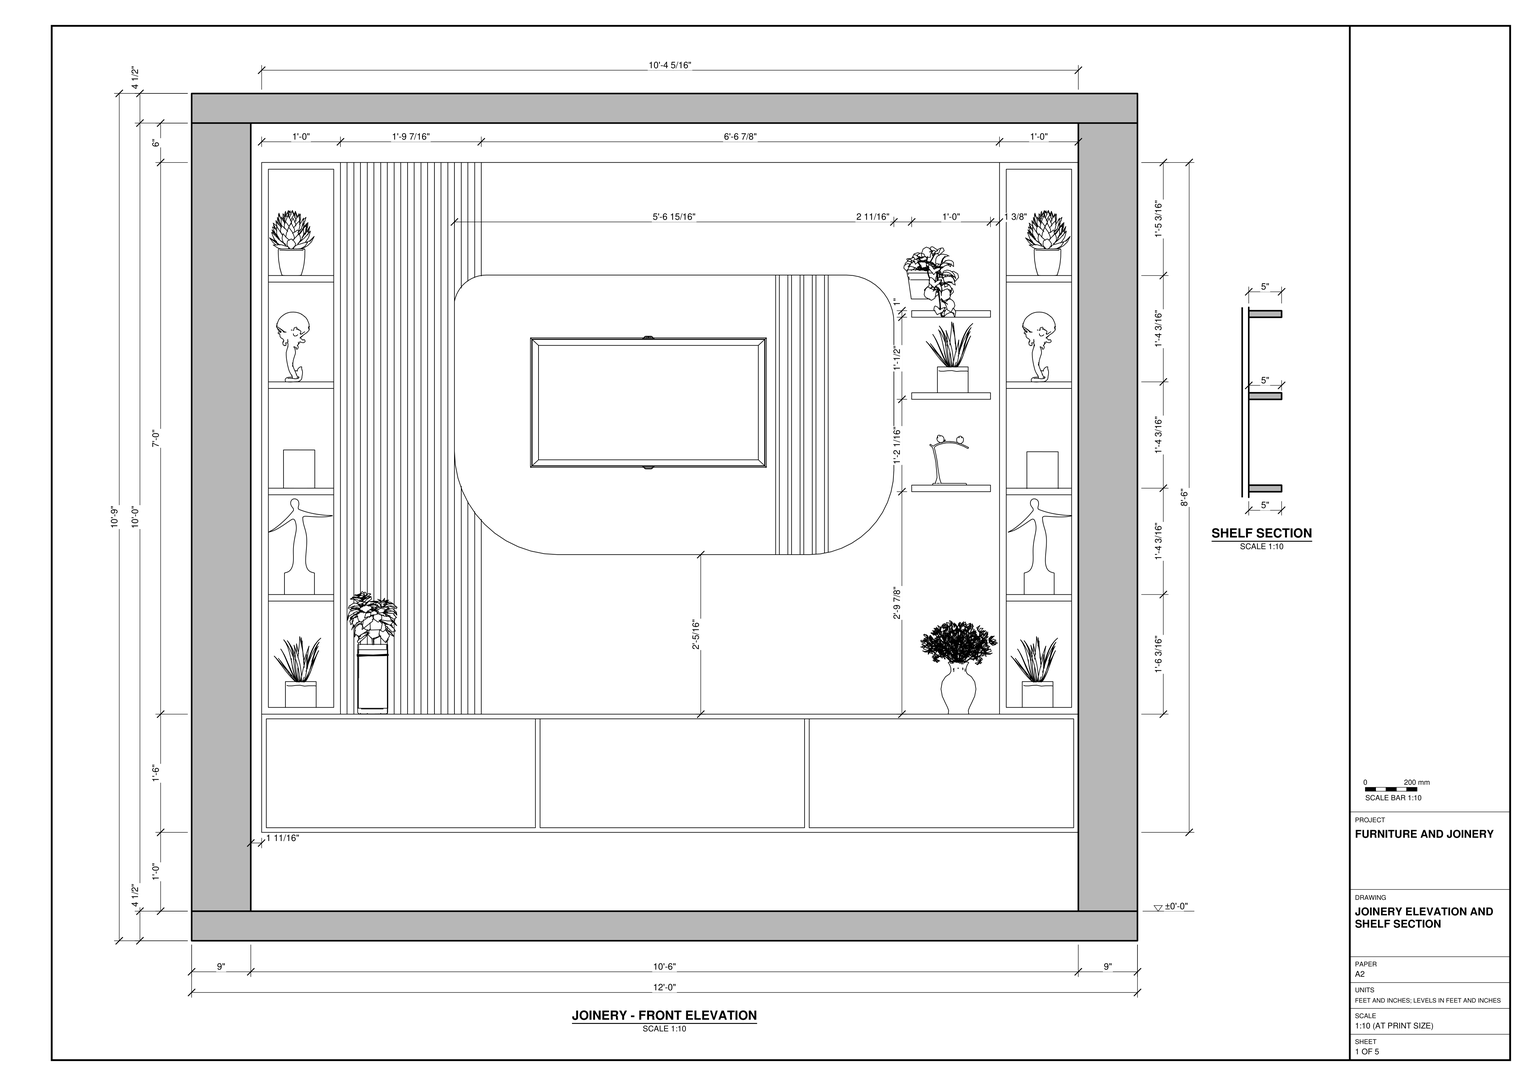
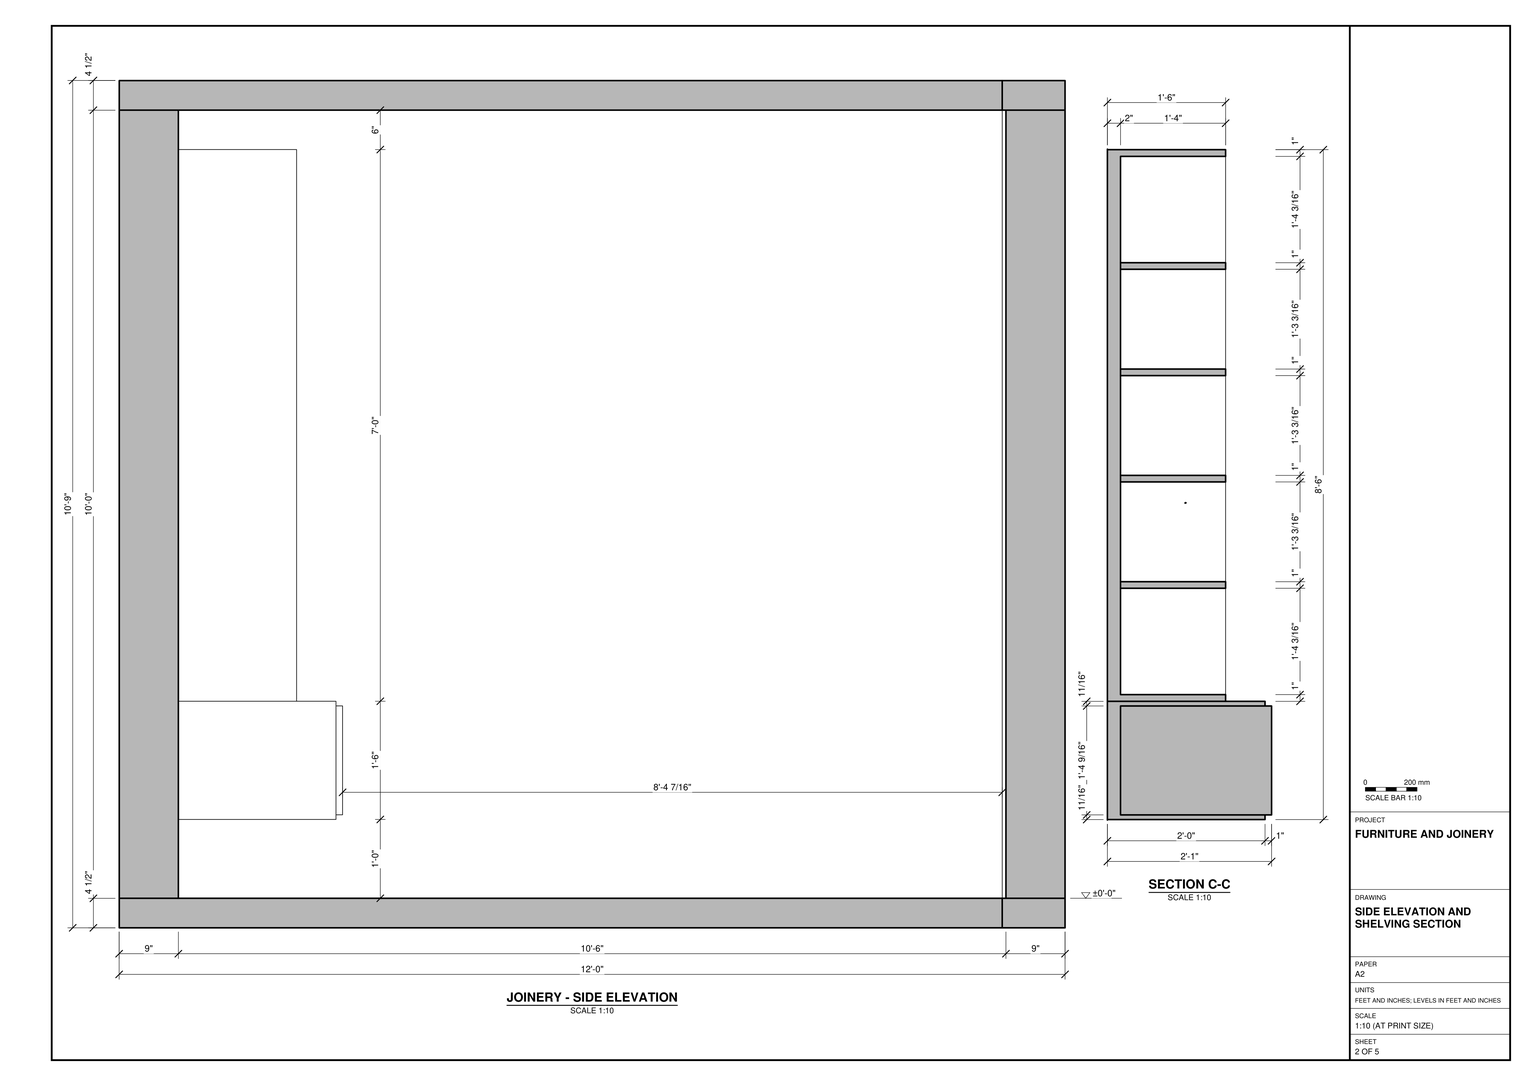
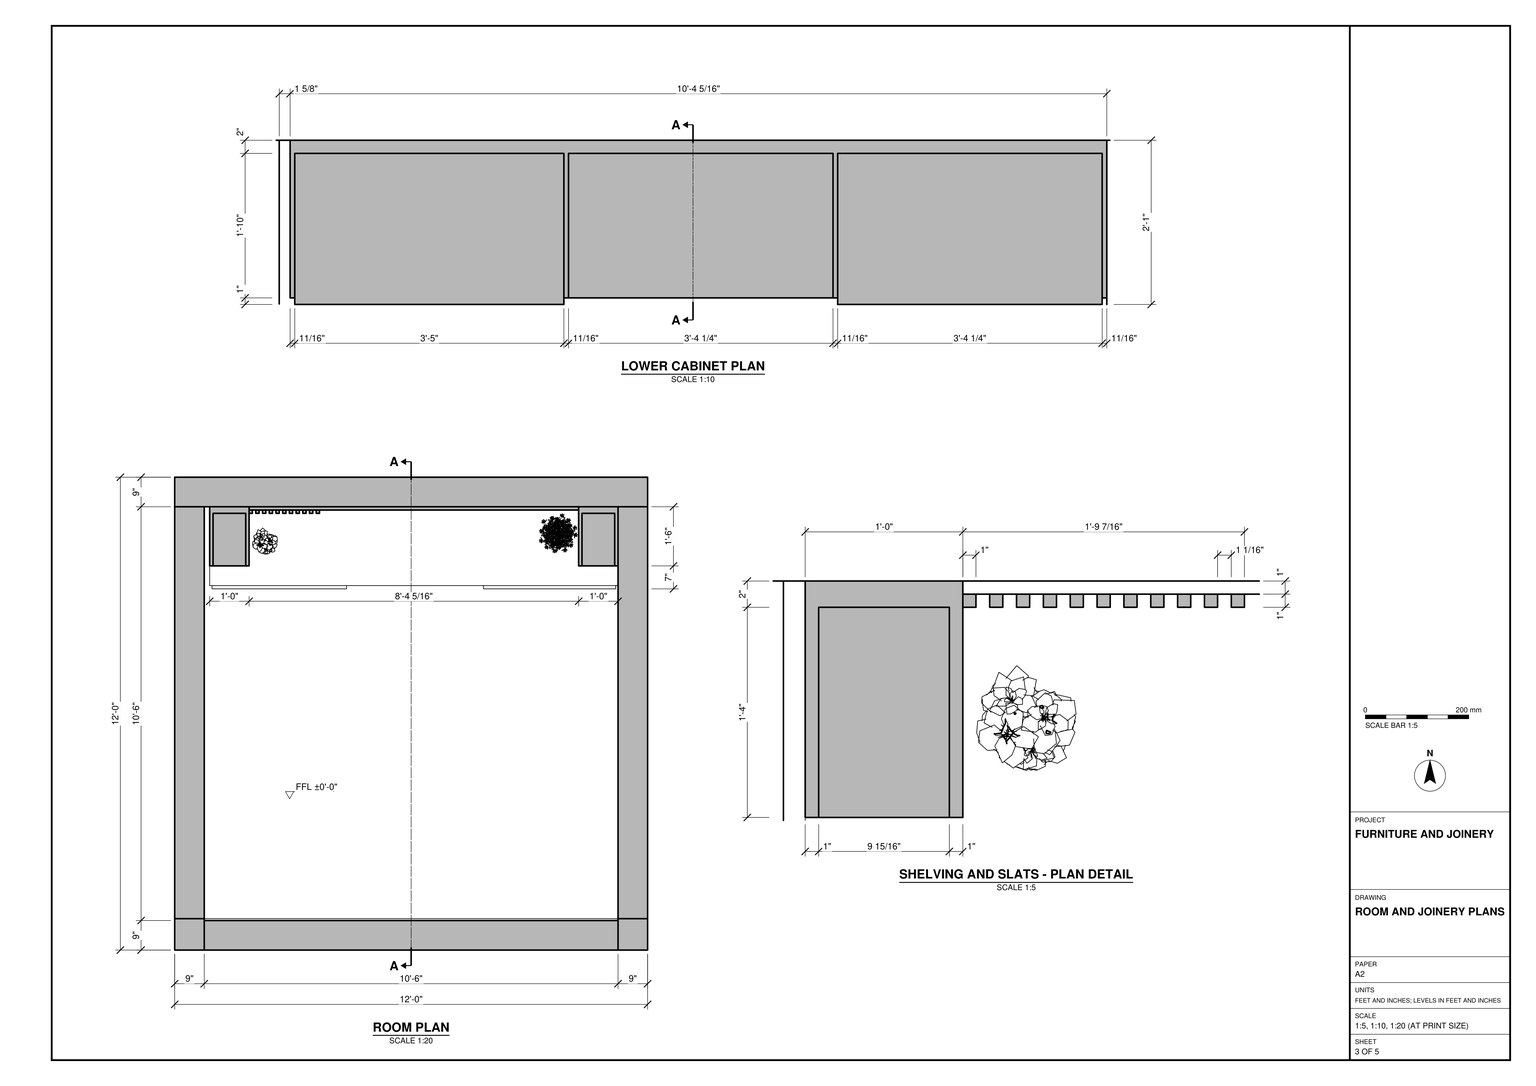
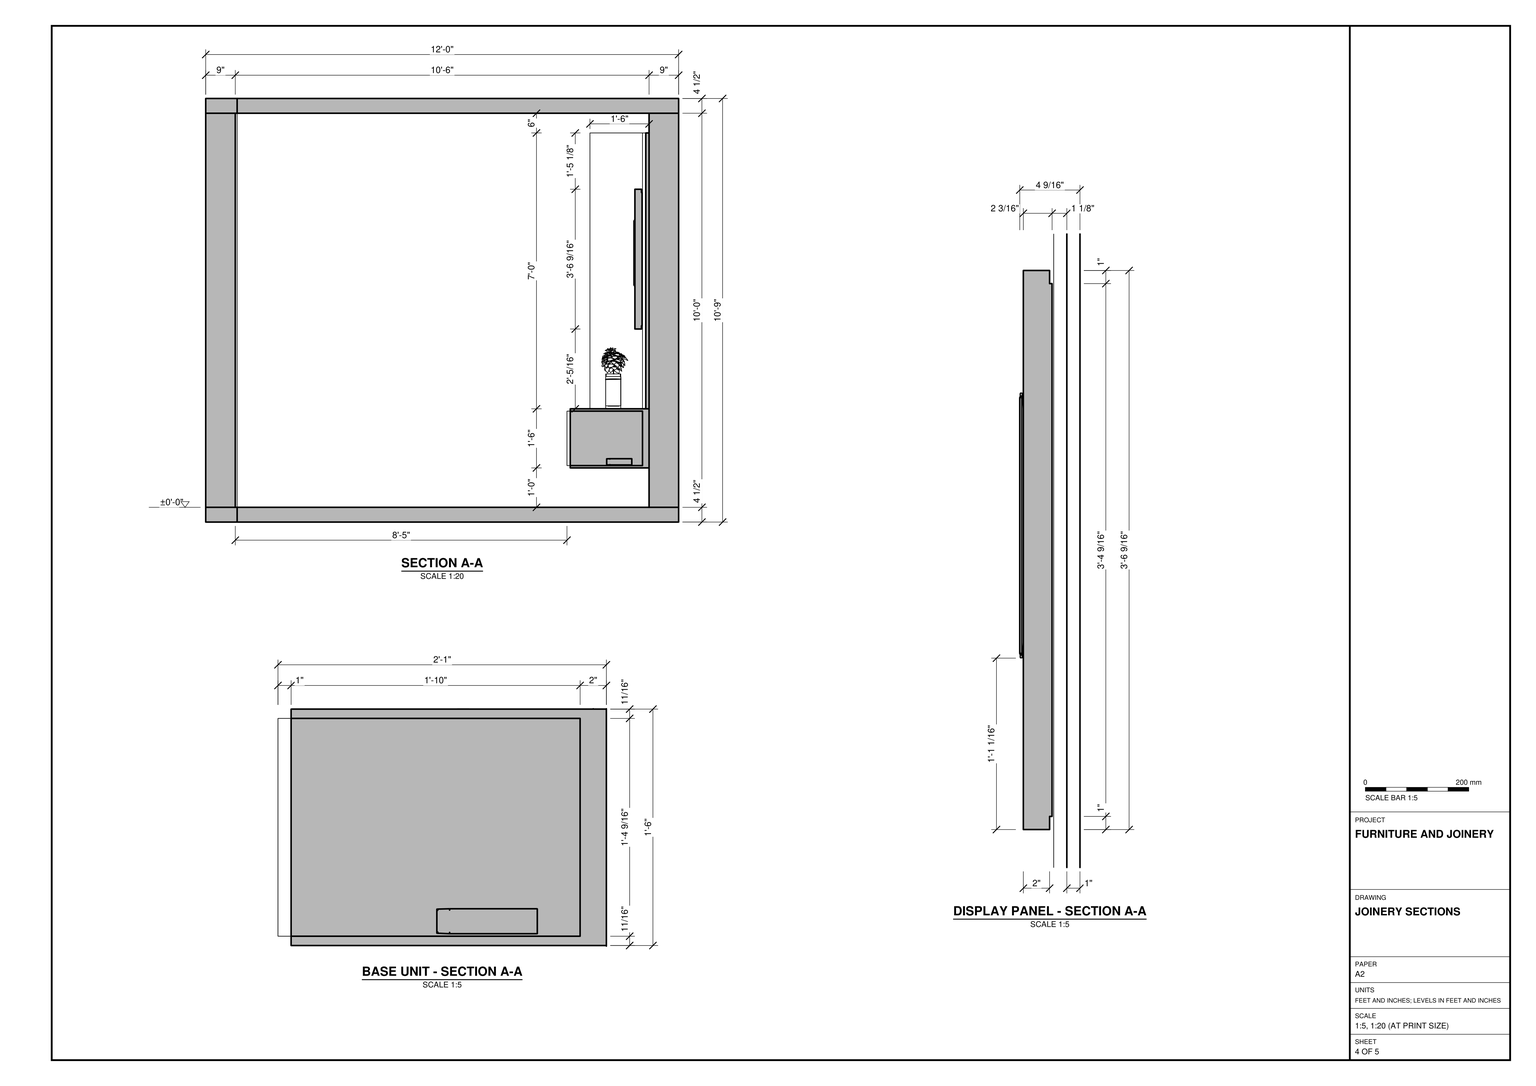
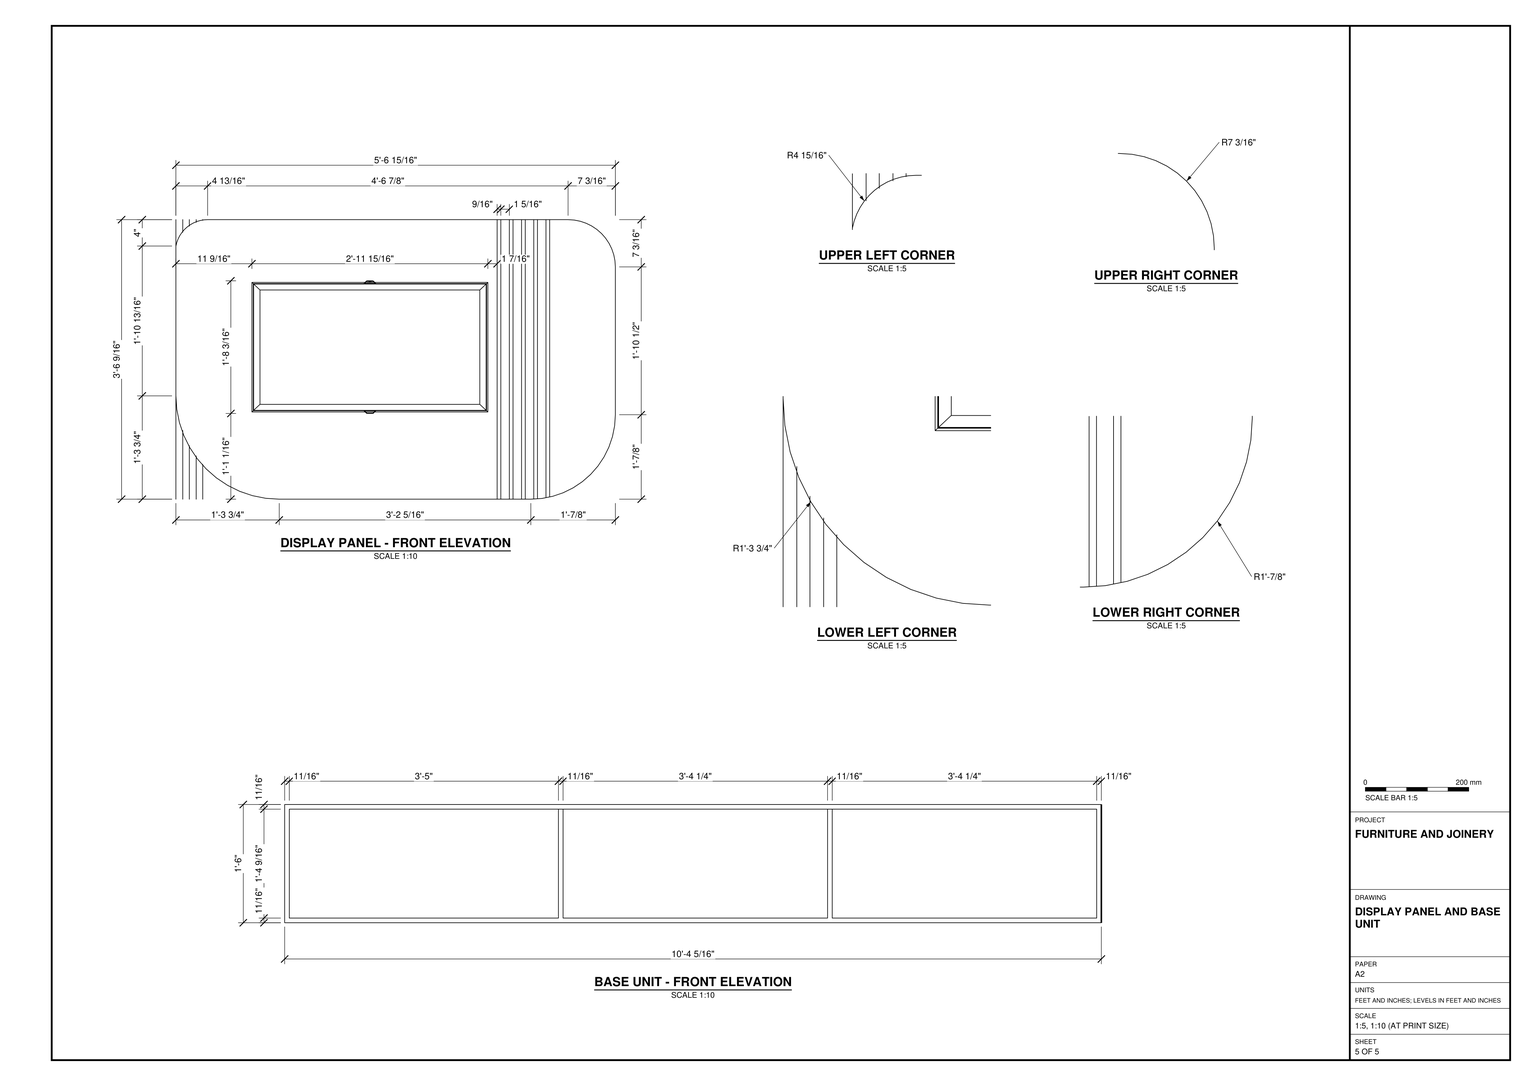
Build the TV wall unit and its enclosing room in SketchUp from task_files/diagram_01.pdf. Work in feet and inches. The room measures 12'-0" by 12'-0" outside the walls and 10'-9" high overall. Set the finished floor at ±0'-0". Model the 9" perimeter walls and the 4 1/2" floor and ceiling slabs, leaving a clear internal height of 10'-0".

Mount the lower cabinet along the wall shown in plan, with its underside 1'-0" above the finished floor. Use the lower cabinet plan and shelving section to set out the three bays and the projection of the outer fronts. Place an open shelving tower at each end of the cabinet. Between the towers, model the broad field of vertical slats beside the left tower and the rounded TV backing panel that overlaps it. Include the narrow slatted strip on the face of the panel. Mount the screen as shown and place three short shelves between the panel and the right tower. Decor and loose items, including the plants and display objects on the shelves and cabinet top, may be any suitable library components.

Keep the walls and slabs and each furniture or joinery piece in separate groups or components, and use components for repeated parts such as slats and shelves. Save one SketchUp model as output_files/wall_mounted_tv_cabinet_with_slatted_panels.skp.

# SketchUp Ruby script. Lengths in inches.
U = 1.inch
M = Sketchup.active_model
def pt(a) = Geom::Point3d.new(a.map { |v| v * U })
def face(e, loops, mat)
  f = e.add_face(loops[0].map { |a| pt(a) })
  loops[1..].each { |l| e.add_face(l.map { |a| pt(a) }).erase! }
  f.material = f.back_material = mat if mat
  f
end
# faces: each face lists its corners as indices into pts; further lists are holes
def faces(e, pts, list, mat = nil) = list.each { |f| face(e, (f[0].is_a?(Array) ? f : [f]).map { |l| l.map { |i| pts[i] } }, mat) }
# xy, xz, yz: faces in a plane at the given z, y or x. An outline is a flat list of corners, or four numbers for a rectangle; further outlines are holes
def ring(l) = l.size == 4 ? [[l[0], l[1]], [l[2], l[1]], [l[2], l[3]], [l[0], l[3]]] : l.each_slice(2).to_a
def flat(e, list, mat, &to3) = list.each { |f| face(e, (f[0].is_a?(Array) ? f : [f]).map { |l| ring(l).map { |u, v| to3.(u, v) } }, mat) }
def xy(e, z, list, mat = nil) = flat(e, list, mat) { |x, y| [x, y, z] }
def xz(e, y, list, mat = nil) = flat(e, list, mat) { |x, z| [x, y, z] }
def yz(e, x, list, mat = nil) = flat(e, list, mat) { |y, z| [x, y, z] }
def lines(e, pts, list) = list.each { |a, b| e.add_line(pt(pts[a]), pt(pts[b])) }
# prism: a flat outline (further loops are holes) pulled along v
def prism(e, loops, v, mat = nil)
  f = face(e, loops, mat); d = Geom::Vector3d.new(v.map { |x| x * U })
  f.pushpull(f.normal.samedirection?(d) ? d.length : -d.length)
end
def box(e, o, s, mat = nil) = prism(e, [[o, [o[0] + s[0], o[1], o[2]], [o[0] + s[0], o[1] + s[1], o[2]], [o[0], o[1] + s[1], o[2]]]], [0, 0, s[2]], mat)
def at(x, y, z, deg = 0) = Geom::Transformation.translation(pt([x, y, z])) * Geom::Transformation.rotation(ORIGIN, Z_AXIS, deg.degrees)
def axes(o, x, y, z) = Geom::Transformation.new([*x, 0, *y, 0, *z, 0, *pt(o).to_a, 1])
def part(name) = M.definitions.add(name)
# library, detail: a bought-in or finely detailed component or shape, given as its bounding box
def library(name, o, s) = part(name).tap { |d| box(d.entities, o, s) }
def detail(e, o, s) = box(e.add_group.entities, o, s)
def put(e, d, t, mat = nil) = e.add_instance(d, t).tap { |i| i.material = mat if mat }
def group(e, t, mat = nil) = e.add_group.tap { |g| g.transformation = t; g.material = mat if mat }.entities
root = M.entities
M.materials.add("Marble White 501 36.79cm").color = [255, 255, 255]
M.materials.add("Pearl Cream 2cm").color = [199, 183, 163]
M.materials.add("Wood 13-11 100cm").color = [206, 162, 102]
M.materials.add("[Translucent Glass Gray]").color = [128, 128, 128]
M.materials["[Translucent Glass Gray]"].alpha = 0.5
c1 = part("Shelf panel")
box(c1.entities,[0,0,0],[9.95,16,1])
c2 = part("Shelf panel \#1")
box(c2.entities,[0,0,0],[12,5,1])
c3 = part("Group13\#1")
p = [[0,0,0],[0,0,-2.18],[-0.76,0,-2.18],[4.97,-2.09,0],[-4.97,-2.09,0],[4.97,2.09,0],
  [4.97,0,0],[-4.97,2.09,0],[0.76,0,-2.18],[-4.97,0,0],[0,0,-3.53]]
lines(c3.entities,p,[[0,1],[1,2],[3,4],[5,6],[7,5],[1,8],[9,0],[0,6],[8,10],[4,9],[6,3],[2,10],
  [9,7]])
c4 = part("Rectangle Light")
put(c4.entities,c3,at(0,0,0))
c5 = part("Group15\#1")
p = [[0,0,0],[0,0,-2.29],[-0.76,0,-2.29],[4.97,-2.43,0],[-4.97,-2.43,0],[4.97,2.43,0],
  [4.97,0,0],[-4.97,2.43,0],[0.76,0,-2.29],[-4.97,0,0],[0,0,-3.7]]
lines(c5.entities,p,[[0,1],[1,2],[3,4],[5,6],[7,5],[1,8],[9,0],[0,6],[8,10],[4,9],[6,3],[2,10],
  [9,7]])
c6 = part("Rectangle Light\#1")
put(c6.entities,c5,at(0,0,0))
c7 = part("Group17\#1")
p = [[0,0,0],[0,0,-2.25],[-0.76,0,-2.25],[4.97,-2.32,0],[-4.97,-2.32,0],[4.97,2.32,0],
  [4.97,0,0],[-4.97,2.32,0],[0.76,0,-2.25],[-4.97,0,0],[0,0,-3.65]]
lines(c7.entities,p,[[0,1],[1,2],[3,4],[5,6],[7,5],[1,8],[9,0],[0,6],[8,10],[4,9],[6,3],[2,10],
  [9,7]])
c8 = part("Rectangle Light\#2")
put(c8.entities,c7,at(0,0,0))
c9 = part("Group19\#1")
p = [[0,0,0],[0,0,-2.1],[-0.76,0,-2.1],[4.97,-1.82,0],[-4.97,-1.82,0],[4.97,1.82,0],
  [4.97,0,0],[-4.97,1.82,0],[0.76,0,-2.1],[-4.97,0,0],[0,0,-3.4]]
lines(c9.entities,p,[[0,1],[1,2],[3,4],[5,6],[7,5],[1,8],[9,0],[0,6],[8,10],[4,9],[6,3],[2,10],
  [9,7]])
c10 = part("Rectangle Light\#3")
put(c10.entities,c9,at(0,0,0))
c11 = part("Group21\#1")
p = [[0,0,0],[0,0,-2.77],[-0.76,0,-2.77],[4.97,-4,0],[-4.97,-4,0],[4.97,4,0],
  [4.97,0,0],[-4.97,4,0],[0.76,0,-2.77],[-4.97,0,0],[0,0,-4.49]]
lines(c11.entities,p,[[0,1],[1,2],[3,4],[5,6],[7,5],[1,8],[9,0],[0,6],[8,10],[4,9],[6,3],[2,10],
  [9,7]])
c12 = part("Rectangle Light\#4")
put(c12.entities,c11,at(0,0,0))
c13 = part("Group23\#1")
p = [[0,0,0],[0,0,-1.9375],[-0.76,0,-1.9375],[4.97,-1.3,0],[-4.97,-1.3,0],[4.97,1.3,0],
  [4.97,0,0],[-4.97,1.3,0],[0.76,0,-1.9375],[-4.97,0,0],[0,0,-3.14]]
lines(c13.entities,p,[[0,1],[1,2],[3,4],[5,6],[7,5],[1,8],[9,0],[0,6],[8,10],[4,9],[6,3],[2,10],
  [9,7]])
c14 = part("Rectangle Light\#5")
put(c14.entities,c13,at(0,0,0))
c15 = part("Group25\#1")
p = [[0,0,0],[0,0,-2.77],[-0.76,0,-2.77],[4.97,-4,0],[-4.97,-4,0],[4.97,4,0],
  [4.97,0,0],[-4.97,4,0],[0.76,0,-2.77],[-4.97,0,0],[0,0,-4.49]]
lines(c15.entities,p,[[0,1],[1,2],[3,4],[5,6],[7,5],[1,8],[9,0],[0,6],[8,10],[4,9],[6,3],[2,10],
  [9,7]])
c16 = part("Rectangle Light\#6")
put(c16.entities,c15,at(0,0,0))
c17 = part("Group27\#1")
p = [[0,0,0],[0,0,-2.77],[-0.76,0,-2.77],[4.97,-4,0],[-4.97,-4,0],[4.97,4,0],
  [4.97,0,0],[-4.97,4,0],[0.76,0,-2.77],[-4.97,0,0],[0,0,-4.49]]
lines(c17.entities,p,[[0,1],[1,2],[3,4],[5,6],[7,5],[1,8],[9,0],[0,6],[8,10],[4,9],[6,3],[2,10],
  [9,7]])
c18 = part("Rectangle Light\#7")
put(c18.entities,c17,at(0,0,0))
c19 = part("Group29\#1")
p = [[0,0,0],[0,0,-2.42],[-0.76,0,-2.42],[4.97,-2.87,0],[-4.97,-2.87,0],[4.97,2.87,0],
  [4.97,0,0],[-4.97,2.87,0],[0.76,0,-2.42],[-4.97,0,0],[0,0,-3.92]]
lines(c19.entities,p,[[0,1],[1,2],[3,4],[5,6],[7,5],[1,8],[9,0],[0,6],[8,10],[4,9],[6,3],[2,10],
  [9,7]])
c20 = part("Rectangle Light\#8")
put(c20.entities,c19,at(0,0,0))
c21 = part("Group31\#1")
p = [[0,0,0],[0,0,-2.77],[-0.76,0,-2.77],[4.97,-4,0],[-4.97,-4,0],[4.97,4,0],
  [4.97,0,0],[-4.97,4,0],[0.76,0,-2.77],[-4.97,0,0],[0,0,-4.49]]
lines(c21.entities,p,[[0,1],[1,2],[3,4],[5,6],[7,5],[1,8],[9,0],[0,6],[8,10],[4,9],[6,3],[2,10],
  [9,7]])
c22 = part("Rectangle Light\#9")
put(c22.entities,c21,at(0,0,0))
c23 = part("Group33\#1")
p = [[0,0,0],[0,0,-2.01],[-0.92,0,-2.01],[6,-0.5,0],[-6,-0.5,0],[6,0.5,0],
  [6,0,0],[-6,0.5,0],[0.92,0,-2.01],[-6,0,0],[0,0,-3.25]]
lines(c23.entities,p,[[0,1],[1,2],[3,4],[5,6],[7,5],[1,8],[9,0],[0,6],[8,10],[4,9],[6,3],[2,10],
  [9,7]])
c24 = part("Rectangle Light\#10")
put(c24.entities,c23,at(0,0,0))
c25 = part("Group35\#1")
p = [[0,0,0],[0,0,-2.01],[-0.92,0,-2.01],[6,-0.5,0],[-6,-0.5,0],[6,0.5,0],
  [6,0,0],[-6,0.5,0],[0.92,0,-2.01],[-6,0,0],[0,0,-3.25]]
lines(c25.entities,p,[[0,1],[1,2],[3,4],[5,6],[7,5],[1,8],[9,0],[0,6],[8,10],[4,9],[6,3],[2,10],
  [9,7]])
c26 = part("Rectangle Light\#11")
put(c26.entities,c25,at(0,0,0))
c27 = part("Group37\#1")
p = [[0,0,0],[0,0,-2.24],[-0.92,0,-2.24],[6,-1.25,0],[-6,-1.25,0],[6,1.25,0],
  [6,0,0],[-6,1.25,0],[0.92,0,-2.24],[-6,0,0],[0,0,-3.625]]
lines(c27.entities,p,[[0,1],[1,2],[3,4],[5,6],[7,5],[1,8],[9,0],[0,6],[8,10],[4,9],[6,3],[2,10],
  [9,7]])
c28 = part("Rectangle Light\#12")
put(c28.entities,c27,at(0,0,0))
c29 = part("Group39\#1")
p = [[0,0,0],[0,0,-19.74],[-9.55,0,-19.74],[62.17,-1.75,0],[-62.17,-1.75,0],[62.17,1.75,0],
  [62.17,0,0],[-62.17,1.75,0],[9.55,0,-19.74],[-62.17,0,0],[0,0,-31.96]]
lines(c29.entities,p,[[0,1],[1,2],[3,4],[5,6],[7,5],[1,8],[9,0],[0,6],[8,10],[4,9],[6,3],[2,10],
  [9,7]])
c30 = part("Rectangle Light\#13")
put(c30.entities,c29,at(0,0,0))
c31 = library("Flat screen television",[0,1.41,1.14],[35.92,0.28,20.21])
c32 = library("Decoration 111 063",[-2.51,-1.28,-0.03],[5.02,2.53,10.66])
c33 = library("Potted Plant 50-23",[-3.4,-3.5,0],[6.8,7,9.93])
c34 = library("Sculpture 108-23",[-12.84,-6.01,0],[25.68,12.02,38.36])
c35 = library("Potted Succulent 003",[-4.09,-3.62,0],[7.1,6.83,10.79])
c36 = library("Potted Basil 50-07",[-3.85,-3.53,0.03],[7.56,8,18.65])
c37 = library("Vase Flowers 26-02",[-5.76,-5.9,0],[11.73,12.02,14.27])
c38 = part("Picture 287 007 003")
xz(c38.entities,-0.14,[[-0.42,-10.51,-0.48,1.54,-8.4,-0.47],[-0.42,-10.51,8.4,-0.625,-0.48,1.54],[8.4,-0.625,0.42,10.51,-0.48,1.54],[-8.4,-0.47,-0.48,1.54,0.42,10.51]])
xz(c38.entities,0.15,[[-9.53,-0.61,-8.62,10.68,-8.59,0.41]])
p = [[-9.66,-0.48,11.82],[-9.67,-0.47,-11.82],[-9.54,-0.5625,0.33],[9.69,-0.45,-11.82],[-0.45,-0.5625,-11.68],[-9.2,-0.42,-11.33],
  [-9.38,-0.56,-0.97],[9.43,-0.59,-11.5625],[9.54,-0.5625,-0.21],[9.66,-0.48,11.8],[-9.65,0.13,-11.74],[9.68,-0.01,-11.84],
  [-9.6875,0.03,11.82],[9.61,0.14,11.72],[8.57,0.13,-10.72],[9.53,0.15,0.45],[-1.36,-0.5625,-11.52],[-9.53,0.15,-0.61],
  [-8.55,0.125,-10.71],[0.76,0.15,-10.77],[9.03,-0.4,-11.22],[9.38,-0.56,-1.28],[-9.15,-0.44,11.29],[-8.7,-0.26,-10.83],
  [-8.98,-0.4,-0.02],[1.39,-0.4,-11.12],[9.2,-0.42,11.32],[-0.87,-0.24,-10.77],[8.42,-0.17,-10.57],[8.73,-0.28,0.95],
  [8.98,-0.4,1.43],[-8.74,-0.28,-1.35],[-0.42,-0.14,-10.51],[-8.4,-0.14,-0.47],[1.32,-0.02,-10.5],[-8.35,-0.02,-0.63],
  [-8.59,0.15,0.41],[-0.78,-0.03,0.125],[8.35,-0.02,0.05],[8.59,0.15,0.53],[8.4,-0.14,-0.625],[9.43,-0.59,11.57],
  [-8.43,-0.17,10.58],[0.42,-0.14,10.51],[8.69,-0.26,10.83],[-8.62,0.15,10.68],[-2.79,-0.02,10.5],[8.58,0.14,10.74],
  [-0.59,-0.24,10.77],[0.07,0.15,10.77],[0.33,-0.4,11.12],[-0.07,-0.5625,11.68],[-0.66,-0.5625,11.52],[-0.01,-0.07,11.85]]
faces(c38.entities,p,[[0,1,2],[1,3,4],[5,1,4],[6,2,1],[1,5,6],[4,3,7],[7,3,8],[8,3,9],
  [1,10,11],[10,1,12],[12,1,0],[1,11,3],[9,3,13],[3,11,13],[11,10,14],[11,14,15],
  [13,11,15],[5,4,16],[16,4,7],[17,10,12],[18,10,17],[18,19,10],[14,10,19],[16,7,20],
  [20,7,21],[21,7,8],[20,5,16],[6,5,22],[5,23,24],[23,5,25],[5,24,22],[25,5,20],
  [21,26,20],[27,20,28],[20,27,25],[28,20,29],[29,20,30],[30,20,26],[27,23,25],[24,23,31],
  [23,27,32],[33,23,32],[31,23,33],[32,27,28],[34,19,18],[14,19,34],[35,18,36],[18,35,37],
  [37,34,18],[14,34,37],[38,14,37],[39,14,38],[36,18,17],[15,14,39],[40,28,29],[32,28,40],
  [26,21,41],[21,8,41],[24,31,22],[22,31,42],[31,33,42],[2,6,22],[43,40,44],[44,40,29],
  [45,17,12],[35,36,45],[35,45,46],[46,37,35],[42,33,43],[41,8,9],[47,37,46],[38,37,47],
  [39,38,47],[22,0,2],[47,15,39],[13,15,47],[44,29,30],[44,30,26],[48,43,44],[42,43,48],
  [49,46,45],[47,46,49],[22,42,48],[13,45,12],[49,45,13],[47,49,13],[22,48,50],[48,44,50],
  [50,44,26],[22,50,26],[0,22,51],[22,52,51],[22,26,52],[52,26,41],[51,52,41],[51,41,9],
  [0,51,9],[9,13,53],[13,12,53],[53,12,0],[9,53,0]])
c39 = library("Plant 260 031 02",[-5.66,-10.61,-5.67],[17.04,23.05,21.91])
c40 = library("Birds Figure 37-23",[-6.28,-2.57,0],[12.56,5.14,16.19])
c41 = library("skpE36B",[-3.84,-2.73,0],[7.68,5.46,1.59])
c42 = part("Group\#1")
box(c42.entities,[0,0,0],[144,144,4.5])
c43 = library("Group\#8",[0,0,0],[66.91,2.1875,42.5625])
c44 = part("Group76\#1")
xz(c44.entities,16.33,[[6.35,0,150.35,4.5]])
c45 = part("Group78\#1")
xz(c45.entities,16.33,[[141.35,4.5,150.35,124.5]])
c46 = part("Group198\#1")
xz(c46.entities,16.33,[[6.35,4.5,15.35,124.5]])
c47 = part("Group202\#1")
xz(c47.entities,16.33,[[6.35,124.5,150.35,129]])
c48 = part("Group73\#1")
put(c48.entities,c44,at(0,0,0))
put(c48.entities,c45,at(0,0,0))
put(c48.entities,c46,at(0,0,0))
put(c48.entities,c47,at(0,0,0))
xy(root,34.5,[[10.66,117,22.66,135],[22.66,133,23.66,134],[24.7,133,25.7,134],[26.74,133,27.74,134],[28.79,133,29.79,134],
  [30.83,133,31.83,134],[32.875,133,33.875,134],[34.92,133,35.92,134],[36.96,133,37.96,134],[39.01,133,40.01,134],
  [41.05,133,42.05,134],[43.09,133,44.09,134],[22.66,134,123,135]])
xy(root,35.53,[[11.68,117,21.63,133]],"Pearl Cream 2cm")
xy(root,117.47,[[11.68,117,21.63,133]])
xy(root,118.5,[[22.66,134,123,135]])
xy(root,118.5,[[10.66,117,22.66,135]],"Pearl Cream 2cm")
xy(root,118.5,[[22.66,133,23.66,134],[24.7,133,25.7,134],[26.74,133,27.74,134],[28.79,133,29.79,134],[30.83,133,31.83,134],
  [32.875,133,33.875,134],[34.92,133,35.92,134],[36.96,133,37.96,134],[39.01,133,40.01,134],[41.05,133,42.05,134],
  [43.09,133,44.09,134]],"Wood 13-11 100cm")
xz(root,117,[[[10.66,34.5,22.66,118.5],[11.68,35.53,21.63,117.47]]],"Pearl Cream 2cm")
xz(root,133,[[11.68,35.53,21.63,117.47]])
xz(root,134,[[44.09,34.5,123,118.5]])
yz(root,10.66,[[117,34.5,135,118.5]],"Pearl Cream 2cm")
yz(root,11.68,[[117,35.53,133,117.47]],"Pearl Cream 2cm")
yz(root,21.63,[[117,35.53,133,117.47]],"Pearl Cream 2cm")
yz(root,22.66,[[117,34.5,133,118.5]],"Pearl Cream 2cm")
yz(root,123,[[134,34.5,135,118.5]])
put(root,c1,at(124.03,117,51.72),"Pearl Cream 2cm")
put(root,c1,at(11.68,117,51.72),"Pearl Cream 2cm")
put(root,c1,at(124.03,117,67.91),"Pearl Cream 2cm")
put(root,c1,at(11.68,117,67.91),"Pearl Cream 2cm")
put(root,c1,at(124.03,117,84.09),"Pearl Cream 2cm")
put(root,c1,at(11.68,117,84.09),"Pearl Cream 2cm")
put(root,c1,at(124.03,117,100.28),"Pearl Cream 2cm")
put(root,c1,at(11.68,117,100.28),"Pearl Cream 2cm")
put(root,c2,at(109.625,129,68.375))
put(root,c2,at(109.625,129,82.4375))
put(root,c2,at(109.625,129,94.9375))
put(root,c4,axes([16.66,130.91,117.46],[1,0,0],[0,-1,0],[0,0,0.43]))
put(root,c6,axes([16.66,130.57,100.27],[1,0,0],[0,-1,0],[0,0,0.38]))
put(root,c8,axes([16.66,130.68,84.08],[1,0,0],[0,-1,0],[0,0,0.46]))
put(root,c10,axes([16.66,131.18,67.9],[1,0,0],[0,-1,0],[0,0,0.51]))
put(root,c12,axes([16.66,129,51.71],[1,0,0],[0,-1,0],[0,0,0.4]))
put(root,c14,axes([129,131.7,117.46],[1,0,0],[0,-1,0],[0,0,0.47]))
put(root,c16,axes([129,129,100.27],[1,0,0],[0,-1,0],[0,0,0.43]))
put(root,c18,axes([129,129,84.08],[1,0,0],[0,-1,0],[0,0,0.33]))
put(root,c20,axes([129,130.13,67.9],[1,0,0],[0,-1,0],[0,0,0.56]))
put(root,c22,axes([129,129,51.71],[1,0,0],[0,-1,0],[0,0,0.5]))
put(root,c24,axes([115.625,133.5,94.93],[1,0,0],[0,-1,0],[0,0,0.4]))
put(root,c26,axes([115.625,133.5,82.43],[1,0,0],[0,-1,0],[0,0,0.41]))
put(root,c28,axes([115.625,132.75,68.37],[1,0,0],[0,-1,0],[0,0,0.3]))
put(root,c30,axes([72.83,133.25,16.49],[1,0,0],[0,-1,0],[0,0,0.11]))
put(root,c31,at(51.58,129,70.7))
put(root,c32,at(129.01,123.56,85.09))
put(root,c32,at(15.43,124.83,85.09))
put(root,c33,at(15.26,124.71,101.28))
put(root,c33,at(130.35,124.51,101.28))
put(root,c34,axes([16.5625,123.09,52.72],[0.38,0,0],[0,0.38,0],[0,0,0.38]))
put(root,c34,axes([129.1875,123.09,52.72],[0.38,0,0],[0,0.38,0],[0,0,0.38]))
put(root,c35,at(16.66,124.33,35.53))
put(root,c35,at(128.84,125.92,35.53))
put(root,c35,at(115.92,132.62,83.4375))
put(root,c36,at(27.5625,124.09,34.5))
put(root,c37,at(116.75,126.8,34.5))
put(root,c38,axes([16.37,121.11,71.82],[-0.2461,0,0],[0,-0.2461,0],[0,0,-0.2461]))
put(root,c38,axes([129.54,126.66,71.55],[-0.2461,0,0],[0,-0.2461,0],[0,0,-0.2461]))
put(root,c39,axes([111.2,128.18,97.72],[0.49,0,0],[0,0.49,0],[0,0,0.49]))
put(root,c40,axes([115.33,132.64,69.375],[0.47,0,0],[0,0.47,0],[0,0,0.47]))
put(root,c41,axes([70.53,125.91,17.08],[1.4,0,0],[0,1.4,0],[0,0,1.4]))
put(root,c42,at(0,0,0))
g1 = group(root,at(135,0,4.5))
box(g1,[0,0,0],[9,135,120])
g2 = group(root,at(123,117,34.5),"Pearl Cream 2cm")
xy(g2,0,[[0,0,12,18]])
xy(g2,1.03,[[1.03,0,10.97,16]])
xy(g2,82.97,[[1.03,0,10.97,16]])
xy(g2,84,[[0,0,12,18]])
xz(g2,0,[[[0,0,12,84],[1.03,1.03,10.97,82.97]]])
xz(g2,16,[[1.03,1.03,10.97,82.97]])
xz(g2,18,[[0,0,12,84]])
yz(g2,0,[[0,0,18,84]])
yz(g2,1.03,[[0,1.03,16,82.97]])
yz(g2,10.97,[[0,1.03,16,82.97]])
yz(g2,12,[[0,0,18,84]])
put(root,c43,at(40.01,130.6875,58.79))
g3 = group(root,at(0,0,4.5))
box(g3,[0,0,0],[9,135,120])
g4 = group(root,at(9,0,4.5))
box(g4,[0,0,0],[126,9,120])
put(root,c42,at(0,0,124.5))
g5 = group(root,at(10.66,111,16.5))
xy(g5,0,[[0,0,124.34,24]])
xy(g5,0.71,[[0.71,-1,41.68,0],[83.37,-1,123.63,0],[0.71,0,41.68,22]])
xy(g5,0.71,[[42.39,0,82.66,22],[83.37,0,123.63,22]],"Wood 13-11 100cm")
xy(g5,17.29,[[0.71,-1,41.68,0],[83.37,-1,123.63,0],[0.71,0,41.68,22],[41.68,0,42.39,22],[82.66,0,83.37,22],
  [83.37,0,123.63,22]])
xy(g5,17.29,[[42.39,0,82.66,22]],"Wood 13-11 100cm")
xy(g5,18,[[0,0,124.34,24]],"Marble White 501 36.79cm")
xz(g5,-1,[[0.71,0.71,41.68,17.29],[83.37,0.71,123.63,17.29]],"Marble White 501 36.79cm")
xz(g5,0,[[[0,0,124.34,18],[0.71,0.71,41.68,17.29],[42.39,0.71,82.66,17.29],[83.37,0.71,123.63,17.29]]])
xz(g5,0,[[42.39,0.71,82.66,17.29]],"[Translucent Glass Gray]")
xz(g5,22,[[0.71,0.71,41.68,17.29]])
xz(g5,22,[[42.39,0.71,82.66,17.29],[83.37,0.71,123.63,17.29]],"Wood 13-11 100cm")
xz(g5,24,[[0,0,124.34,18]])
yz(g5,0,[[0,0,24,18]],"Marble White 501 36.79cm")
yz(g5,0.71,[[-1,0.71,0,17.29],[0,0.71,22,17.29]])
yz(g5,41.68,[[-1,0.71,0,17.29],[0,0.71,22,17.29]])
yz(g5,42.39,[[0,0.71,22,17.29]],"Wood 13-11 100cm")
yz(g5,82.66,[[0,0.71,22,17.29]],"Wood 13-11 100cm")
yz(g5,83.37,[[-1,0.71,0,17.29]])
yz(g5,83.37,[[0,0.71,22,17.29]],"Wood 13-11 100cm")
yz(g5,123.63,[[-1,0.71,0,17.29],[0,0.71,22,17.29]])
yz(g5,124.34,[[0,0,24,18]])
g6 = group(root,at(0,135,4.5))
box(g6,[0,0,0],[144,9,120])
g7 = group(root,at(9,101.14,4.5),"Wood 13-11 100cm")
xz(g7,31.86,[[13.66,30,14.66,114],[15.7,30,16.7,114],[17.74,30,18.74,114],[19.79,30,20.79,114],[21.83,30,22.83,114],
  [23.875,30,24.875,114],[25.92,30,26.92,114],[27.96,30,28.96,114],[30.01,30,31.01,114],[32.05,30,33.05,114],
  [34.09,30,35.09,114]])
xz(g7,32.86,[[13.66,30,14.66,114],[14.66,30,15.7,114],[15.7,30,16.7,114],[16.7,30,17.74,114],[17.74,30,18.74,114],
  [18.74,30,19.79,114],[19.79,30,20.79,114],[20.79,30,21.83,114],[21.83,30,22.83,114],[22.83,30,23.875,114],
  [23.875,30,24.875,114],[24.875,30,25.92,114],[25.92,30,26.92,114],[26.92,30,27.96,114],[27.96,30,28.96,114],
  [28.96,30,30.01,114],[30.01,30,31.01,114],[31.01,30,32.05,114],[32.05,30,33.05,114],[33.05,30,34.09,114],
  [34.09,30,35.09,114]])
xz(g7,33.86,[[1.66,30,13.66,114],[13.66,30,114,114]])
yz(g7,13.66,[[31.86,30,32.86,114],[32.86,30,33.86,114]])
yz(g7,14.66,[[31.86,30,32.86,114]])
yz(g7,15.7,[[31.86,30,32.86,114]])
yz(g7,16.7,[[31.86,30,32.86,114]])
yz(g7,17.74,[[31.86,30,32.86,114]])
yz(g7,18.74,[[31.86,30,32.86,114]])
yz(g7,19.79,[[31.86,30,32.86,114]])
yz(g7,20.79,[[31.86,30,32.86,114]])
yz(g7,21.83,[[31.86,30,32.86,114]])
yz(g7,22.83,[[31.86,30,32.86,114]])
yz(g7,23.875,[[31.86,30,32.86,114]])
yz(g7,24.875,[[31.86,30,32.86,114]])
yz(g7,25.92,[[31.86,30,32.86,114]])
yz(g7,26.92,[[31.86,30,32.86,114]])
yz(g7,27.96,[[31.86,30,32.86,114]])
yz(g7,28.96,[[31.86,30,32.86,114]])
yz(g7,30.01,[[31.86,30,32.86,114]])
yz(g7,31.01,[[31.86,30,32.86,114]])
yz(g7,32.05,[[31.86,30,32.86,114]])
yz(g7,33.05,[[31.86,30,32.86,114]])
yz(g7,34.09,[[31.86,30,32.86,114]])
yz(g7,35.09,[[31.86,30,32.86,114]])
put(root,c48,at(-6.35,-6.77,0))
